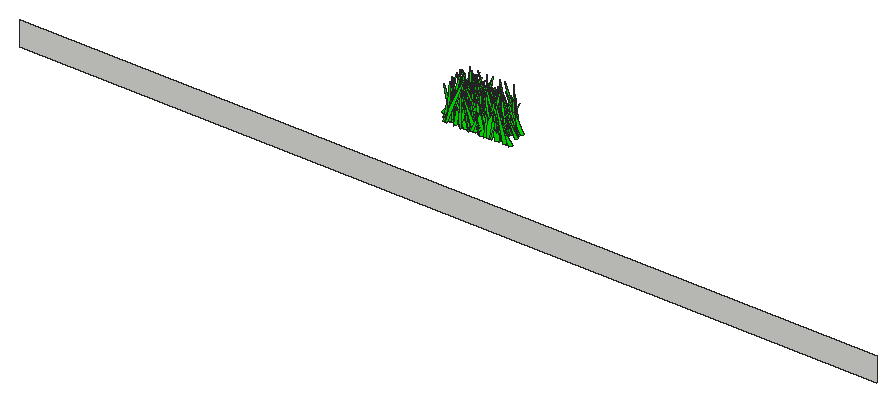
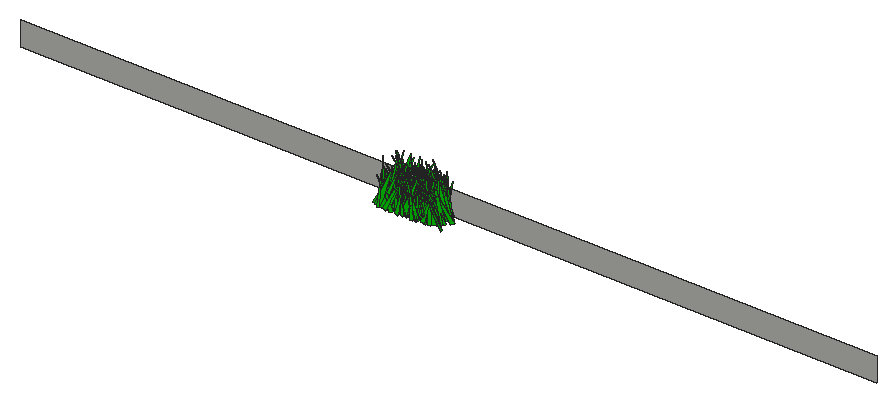
# SketchUp Ruby script. Lengths in inches.
U = 1.inch
M = Sketchup.active_model
def pt(a) = Geom::Point3d.new(a.map { |v| v * U })
def face(e, loops, mat)
  f = e.add_face(loops[0].map { |a| pt(a) })
  loops[1..].each { |l| e.add_face(l.map { |a| pt(a) }).erase! }
  f.material = f.back_material = mat if mat
  f
end
# faces: each face lists its corners as indices into pts; further lists are holes
def faces(e, pts, list, mat = nil) = list.each { |f| face(e, (f[0].is_a?(Array) ? f : [f]).map { |l| l.map { |i| pts[i] } }, mat) }
# xy, xz, yz: faces in a plane at the given z, y or x. An outline is a flat list of corners, or four numbers for a rectangle; further outlines are holes
def ring(l) = l.size == 4 ? [[l[0], l[1]], [l[2], l[1]], [l[2], l[3]], [l[0], l[3]]] : l.each_slice(2).to_a
def flat(e, list, mat, &to3) = list.each { |f| face(e, (f[0].is_a?(Array) ? f : [f]).map { |l| ring(l).map { |u, v| to3.(u, v) } }, mat) }
def xy(e, z, list, mat = nil) = flat(e, list, mat) { |x, y| [x, y, z] }
def xz(e, y, list, mat = nil) = flat(e, list, mat) { |x, z| [x, y, z] }
def yz(e, x, list, mat = nil) = flat(e, list, mat) { |y, z| [x, y, z] }
def lines(e, pts, list) = list.each { |a, b| e.add_line(pt(pts[a]), pt(pts[b])) }
# prism: a flat outline (further loops are holes) pulled along v
def prism(e, loops, v, mat = nil)
  f = face(e, loops, mat); d = Geom::Vector3d.new(v.map { |x| x * U })
  f.pushpull(f.normal.samedirection?(d) ? d.length : -d.length)
end
def box(e, o, s, mat = nil) = prism(e, [[o, [o[0] + s[0], o[1], o[2]], [o[0] + s[0], o[1] + s[1], o[2]], [o[0], o[1] + s[1], o[2]]]], [0, 0, s[2]], mat)
def at(x, y, z, deg = 0) = Geom::Transformation.translation(pt([x, y, z])) * Geom::Transformation.rotation(ORIGIN, Z_AXIS, deg.degrees)
def axes(o, x, y, z) = Geom::Transformation.new([*x, 0, *y, 0, *z, 0, *pt(o).to_a, 1])
def part(name) = M.definitions.add(name)
# library, detail: a bought-in or finely detailed component or shape, given as its bounding box
def library(name, o, s) = part(name).tap { |d| box(d.entities, o, s) }
def detail(e, o, s) = box(e.add_group.entities, o, s)
def put(e, d, t, mat = nil) = e.add_instance(d, t).tap { |i| i.material = mat if mat }
def group(e, t, mat = nil) = e.add_group.tap { |g| g.transformation = t; g.material = mat if mat }.entities
root = M.entities
M.materials.add("[0065_Lime]").color = [0, 255, 0]
c1 = part("fur_instance\#9")
p = [[0.8125,0,1.79],[0.67,-0.02,1.48],[0,-0.11,0],[0,0.11,0]]
faces(c1.entities,p,[[0,1,2,3]])
xz(root,0,[[5.71,-11.8125,282.96,-3.9375]])
put(root,c1,axes([127.84,19.68,1.48],[-1.88355,-0.98454,0.43737],[6.79232,-0.27513,-1.3991],[1.80123,0.00797,5.73327]),"[0065_Lime]")
put(root,c1,axes([127.38,20.51,1.48],[1.59601,1.1704,1.8528],[-8.58809,0.18125,1.05814],[0.89931,-0.34625,6.8167]),"[0065_Lime]")
put(root,c1,axes([130.26,19.51,1.48],[-0.54422,0.77974,1.08313],[-5.57029,-0.03175,-1.08582],[-1.23969,-0.19963,4.40342]),"[0065_Lime]")
put(root,c1,axes([130.34,19.59,1.48],[-0.93781,-0.99188,0.31196],[6.99006,-0.122,0.90495],[-1.05455,0.07338,5.721]),"[0065_Lime]")
put(root,c1,axes([128.24,18.89,1.48],[6.61511,0.29179,0.90941],[-1.22565,0.82503,-2.97163],[-2.01491,0.45612,4.79329]),"[0065_Lime]")
put(root,c1,axes([127.42,23.19,1.48],[5.41493,-0.76132,2.38586],[6.13583,0.71594,-1.55863],[-0.55627,0.48607,6.03266]),"[0065_Lime]")
put(root,c1,axes([127.24,24.58,1.48],[4.29917,0.35555,0.2939],[-2.5389,0.58261,0.95518],[0.29454,-0.16761,3.94368]),"[0065_Lime]")
put(root,c1,axes([129.75,19.5625,1.48],[4.59734,0.95656,1.01862],[-6.47828,0.66904,-1.70752],[-2.43733,0.02601,6.45982]),"[0065_Lime]")
put(root,c1,axes([127.46,20.96,1.48],[6.0247,-0.57137,1.15032],[4.28164,0.83087,-1.00807],[-0.44872,0.25659,5.8257]),"[0065_Lime]")
put(root,c1,axes([127.82,21.4375,1.48],[3.3729,-1.10577,2.71672],[8.5403,0.41349,-1.37583],[0.37891,0.52337,6.8269]),"[0065_Lime]")
put(root,c1,axes([129.15,19.16,1.48],[4.45711,-0.955,0.5882],[6.67866,0.63434,1.02719],[-1.4519,-0.01376,6.53068]),"[0065_Lime]")
put(root,c1,axes([125.68,26.09,1.48],[8.65052,0.43303,0.24417],[-3.03777,1.16273,2.10871],[0.59917,-0.35692,7.16578]),"[0065_Lime]")
put(root,c1,axes([131.32,20.62,1.48],[-0.20186,0.8961,0.26979],[-6.1799,-0.01567,-1.31541],[-1.60837,-0.05226,5.02039]),"[0065_Lime]")
put(root,c1,axes([127.74,20.66,1.48],[4.18471,0.56885,0.97148],[-4.2005,0.53816,1.4123],[0.413,-0.29038,4.52052]),"[0065_Lime]")
put(root,c1,axes([127.03,23.24,1.48],[2.50533,0.82601,1.27648],[-5.75386,0.24416,2.17777],[1.97748,-0.33608,4.71943]),"[0065_Lime]")
put(root,c1,axes([130.07,21.78,1.48],[6.79954,-0.91936,0.33816],[5.63027,0.86202,3.62678],[-3.35854,-0.41621,6.76457]),"[0065_Lime]")
put(root,c1,axes([125.55,21.65,1.48],[6.99956,-0.64941,0.12769],[4.27451,0.89339,-2.7803],[1.76403,0.41198,6.23041]),"[0065_Lime]")
put(root,c1,axes([130.36,22.59,1.48],[4.44285,-0.90294,1.68025],[6.30472,0.67925,1.20134],[-2.41016,0.11237,6.23995]),"[0065_Lime]")
put(root,c1,axes([129.98,25.67,1.48],[-3.74509,-0.71683,0.72348],[4.77236,-0.53765,-1.5054],[2.00987,-0.05907,4.92262]),"[0065_Lime]")
put(root,c1,axes([132.24,25.77,1.48],[-5.1,-0.70608,1.60563],[5.3946,-0.68136,1.29688],[0.21005,0.35533,5.67745]),"[0065_Lime]")
put(root,c1,axes([131.05,18.73,1.48],[6.55752,0.35829,2.1421],[-1.00498,0.90507,-3.03712],[-3.52512,0.40847,4.85064]),"[0065_Lime]")
put(root,c1,axes([127.3,20.04,1.48],[5.74238,1.05461,0.23828],[-7.4017,0.78577,1.48494],[1.27591,-0.18803,7.54194]),"[0065_Lime]")
put(root,c1,axes([131.45,21.28,1.48],[-7.5349,0.65973,1.91206],[-4.4009,-1.10865,1.34334],[2.86371,0.03211,7.09539]),"[0065_Lime]")
put(root,c1,axes([132.42,23.52,1.48],[3.62252,-0.92289,3.16381],[7.00436,0.64235,0.97245],[-3.03373,0.38107,6.02306]),"[0065_Lime]")
put(root,c1,axes([132.51,24.68,1.48],[-7.99573,0.44902,0.72866],[-2.3719,-1.00287,3.48749],[2.32107,0.52195,6.07398]),"[0065_Lime]")
put(root,c1,axes([135.23,25.68,1.48],[-4.03532,0.78482,0.32967],[-5.01925,-0.47578,-2.69597],[-2.4831,-0.31369,4.91378]),"[0065_Lime]")
put(root,c1,axes([131.94,25,1.48],[-8.27127,0.40188,1.98698],[-2.09799,-1.18121,2.22707],[3.12169,0.27096,6.76147]),"[0065_Lime]")
put(root,c1,axes([128.33,18.53,1.48],[8.13111,-0.63911,0.90401],[4.67579,1.1246,-1.1847],[-0.24197,0.25518,7.48517]),"[0065_Lime]")
put(root,c1,axes([131.125,19.42,1.48],[3.67897,0.90282,0.57289],[-6.32832,0.5263,-0.90377],[-1.31457,-0.00698,5.95405]),"[0065_Lime]")
put(root,c1,axes([130.91,24.08,1.48],[-3.01179,-0.78076,1.41981],[5.4629,-0.47444,-1.07506],[2.01886,0.11905,5.02715]),"[0065_Lime]")
put(root,c1,axes([132.97,19.4,1.48],[-4.59077,0.4352,1.21307],[-3.40326,-0.62465,-1.01218],[0.48395,-0.26432,4.38935]),"[0065_Lime]")
put(root,c1,axes([133.59,23.83,1.48],[-3.84347,0.70969,0.95469],[-5.16002,-0.50333,-1.20683],[-0.50961,-0.256,5.01942]),"[0065_Lime]")
put(root,c1,axes([134.07,19.27,1.48],[-2.09709,0.67834,0.34016],[-4.55195,-0.25384,-1.60503],[-1.66105,-0.16079,3.96898]),"[0065_Lime]")
put(root,c1,axes([133.15,19.125,1.48],[-5.94132,0.15971,0.73819],[-0.86372,-0.81893,1.33753],[1.17021,0.20643,4.7351]),"[0065_Lime]")
put(root,c1,axes([132.39,21.64,1.48],[6.24431,-0.53352,1.84624],[2.8622,0.90798,2.38724],[-3.37273,-0.21722,5.44403]),"[0065_Lime]")
put(root,c1,axes([131.27,23.78,1.48],[7.11686,0.5597,1.48646],[-3.72566,1.03061,-1.20132],[-2.30748,0.06225,6.52426]),"[0065_Lime]")
put(root,c1,axes([130.68,19.57,1.48],[7.94743,0.52318,0.88197],[-3.31714,1.09713,-2.03117],[-2.00871,0.25819,6.84374]),"[0065_Lime]")
put(root,c1,axes([129.43,24.15,1.48],[8.37788,-0.04501,0.69259],[0.48877,1.15748,-1.39106],[-0.76727,0.24584,6.67627]),"[0065_Lime]")
put(root,c1,axes([131.43,18.84,1.48],[6.79196,0.75194,0.95465],[-5.00898,0.95874,-1.72581],[-2.2188,0.13739,6.81835]),"[0065_Lime]")
put(root,c1,axes([129.02,24.9,1.48],[0.3596,-1.28657,0.19297],[8.49208,0.03434,-2.79914],[3.4311,0.04986,6.90773]),"[0065_Lime]")
put(root,c1,axes([133.03,24.78,1.48],[1.52368,-0.62606,0.68471],[4.2637,0.24029,1.0844],[-1.54267,0.04576,3.67341]),"[0065_Lime]")
put(root,c1,axes([133.73,24.19,1.48],[-2.94012,0.67888,1.28121],[-5.07695,-0.38151,-0.93462],[-0.21714,-0.27226,4.5044]),"[0065_Lime]")
put(root,c1,axes([131.56,25.58,1.48],[5.7235,0.63245,0.26773],[-4.17912,0.77098,-1.91723],[-1.70327,0.23356,5.60375]),"[0065_Lime]")
put(root,c1,axes([133.91,26.06,1.48],[-7.40548,-0.24155,1.73235],[2.13299,-1.05028,1.12575],[1.71492,0.26327,6.08053]),"[0065_Lime]")
put(root,c1,axes([134.16,19.74,1.48],[-5.31076,0.24298,0.03166],[-1.63072,-0.7093,1.42198],[0.57639,0.23198,4.31477]),"[0065_Lime]")
put(root,c1,axes([131.96,22.92,1.48],[-1.17886,0.83181,1.0892],[-5.88421,-0.2036,0.99651],[1.4868,-0.14626,4.80742]),"[0065_Lime]")
put(root,c1,axes([132.56,24.0625,1.48],[-2.37055,0.96935,0.27023],[-6.76377,-0.33583,1.10872],[1.39646,0.01894,5.82882]),"[0065_Lime]")
put(root,c1,axes([134.84,18.94,1.48],[-3.13554,0.64764,0.29956],[-4.55574,-0.42207,-0.97376],[-0.78964,-0.13661,4.42852]),"[0065_Lime]")
put(root,c1,axes([130.73,19.98,1.48],[1.56005,-0.66734,0.73],[4.53678,0.1565,-1.62082],[1.6665,0.19866,3.72907]),"[0065_Lime]")
put(root,c1,axes([132.38,19.88,1.48],[-4.58927,0.68722,1.07387],[-4.29088,-0.66041,2.02906],[2.69252,0.11889,5.06393]),"[0065_Lime]")
put(root,c1,axes([129.71,23.44,1.48],[6.23921,0.88257,0.74493],[-6.29047,0.8357,1.68191],[0.84722,-0.29463,7.00204]),"[0065_Lime]")
put(root,c1,axes([130.44,21.64,1.48],[8.73592,0.02809,1.0369],[-0.69268,1.13637,2.82962],[-1.08864,-0.49762,6.52025]),"[0065_Lime]")
put(root,c1,axes([131.79,22.34,1.48],[5.87142,0.09701,0.89122],[-0.36134,0.80914,-1.3762],[-1.24358,0.22291,4.60766]),"[0065_Lime]")
put(root,c1,axes([131.51,22.72,1.48],[2.46936,-0.62367,0.64679],[4.41968,0.30954,-1.16271],[0.89336,0.19254,3.96441]),"[0065_Lime]")
put(root,c1,axes([130.8,24.49,1.48],[5.97716,-0.62244,1.40996],[4.75421,0.76903,-1.95864],[0.15444,0.41634,5.72576]),"[0065_Lime]")
put(root,c1,axes([136.28,19.59,1.48],[-2.50424,-0.58005,0.30026],[3.56717,-0.27082,2.15339],[-2.10991,0.2306,3.2843]),"[0065_Lime]")
put(root,c1,axes([135.14,25.03,1.48],[1.04984,0.83458,1.67244],[-5.80698,0.24086,-1.61581],[-2.40459,-0.2173,4.63229]),"[0065_Lime]")
put(root,c1,axes([133.13,18.63,1.48],[-4.8097,-0.56357,1.36731],[3.48379,-0.71014,-1.69983],[2.60272,-0.09091,4.80199]),"[0065_Lime]")
put(root,c1,axes([133.46,23.15,1.48],[4.6814,0.82059,0.23858],[-5.52111,0.63774,-1.82309],[-1.92513,0.16646,5.80864]),"[0065_Lime]")
put(root,c1,axes([132.64,24.52,1.48],[5.42971,-0.40406,0.14494],[2.72941,0.73854,1.33857],[-0.9222,-0.19315,4.81511]),"[0065_Lime]")
put(root,c1,axes([136.28,24.37,1.48],[-5.68369,0.11795,0.29079],[-0.90555,-0.76792,-1.27349],[0.1111,-0.22512,4.49647]),"[0065_Lime]")
put(root,c1,axes([134.37,25.72,1.48],[-3.44311,-0.5649,0.56146],[3.80648,-0.4906,-1.09557],[1.46586,-0.05291,4.16373]),"[0065_Lime]")
put(root,c1,axes([131.8,21.55,1.48],[3.70211,-1.08959,0.22756],[7.67112,0.50743,-1.15718],[1.16561,0.12116,6.89284]),"[0065_Lime]")
put(root,c1,axes([134.05,24.375,1.48],[6.28003,-0.35878,2.98637],[3.7125,0.91411,-1.4855],[-2.49312,0.45747,5.31045]),"[0065_Lime]")
put(root,c1,axes([135.52,20.25,1.48],[-7.56193,0.32921,1.29869],[-1.80756,-1.05216,1.97363],[2.18419,0.26903,6.12951]),"[0065_Lime]")
put(root,c1,axes([131.31,20.84,1.48],[8.74302,0.23964,0.05454],[-1.65699,1.2036,-1.46434],[-0.40912,0.24653,7.09621]),"[0065_Lime]")
put(root,c1,axes([134.72,22.1,1.48],[5.09673,-0.77492,1.57839],[5.32278,0.7647,1.20829],[-2.41775,0.04996,5.98742]),"[0065_Lime]")
put(root,c1,axes([133.23,18.88,1.48],[7.89269,-0.3569,2.56838],[3.54797,1.07796,-2.19447],[-1.95783,0.51467,6.37725]),"[0065_Lime]")
put(root,c1,axes([137.68,22.93,1.48],[-5.83603,-0.4904,0.36089],[3.45664,-0.77685,1.61127],[-0.65455,0.27001,5.29127]),"[0065_Lime]")
put(root,c1,axes([137.08,24.58,1.48],[-3.639,0.53306,1.42163],[-4.09878,-0.39308,-2.00284],[-0.8036,-0.40899,3.77784]),"[0065_Lime]")
put(root,c1,axes([133.62,24.89,1.48],[6.8678,-0.07761,1.28988],[0.21147,0.9707,1.21212],[-1.66582,-0.19674,5.47175]),"[0065_Lime]")
put(root,c1,axes([136,18.625,1.48],[-4.96977,-0.14821,1.25753],[1.45572,-0.69353,1.06749],[1.17619,0.23213,3.99226]),"[0065_Lime]")
put(root,c1,axes([137.1,25.68,1.48],[-8.70175,-0.25326,0.94629],[1.23958,-1.15103,-2.78079],[1.7508,-0.44381,6.67205]),"[0065_Lime]")
put(root,c1,axes([133.01,19.67,1.48],[4.3497,-0.27401,0.18043],[1.90095,0.56937,-1.34642],[0.48806,0.22443,3.63611]),"[0065_Lime]")
put(root,c1,axes([136.52,20.64,1.48],[-6.98711,-0.41337,0.98387],[2.65637,-0.984,-1.37157],[1.74944,-0.15684,6.01213]),"[0065_Lime]")
put(root,c1,axes([135.93,19.75,1.48],[2.51291,-0.7947,0.59097],[5.3811,0.36742,1.41693],[-1.8859,-0.01055,4.83042]),"[0065_Lime]")
put(root,c1,axes([135.55,22.21,1.48],[-6.97969,0.72171,2.2043],[-5.02118,-1.04913,0.99068],[2.91733,-0.07903,6.97888]),"[0065_Lime]")
put(root,c1,axes([134.34,23.32,1.48],[6.02519,0.46674,0.69826],[-3.03176,0.83849,-1.47195],[-1.60571,0.16823,5.39932]),"[0065_Lime]")
put(root,c1,axes([137.44,21.26,1.48],[-4.47893,-0.43545,1.21376],[3.42862,-0.53799,1.9036],[-0.27257,0.38812,4.0004]),"[0065_Lime]")
put(root,c1,axes([136.15,22.61,1.48],[-5.37648,-0.31735,1.10742],[2.00376,-0.77406,-0.99633],[1.71433,-0.09052,4.63764]),"[0065_Lime]")
put(root,c1,axes([133.04,22.99,1.48],[8.93321,-0.06221,0.97484],[0.20968,1.24475,1.39025],[-1.26028,-0.23383,7.14124]),"[0065_Lime]")
put(root,c1,axes([133.65,25.9,1.48],[6.77364,-0.5246,1.84911],[4.26715,0.92129,-1.58402],[-0.94702,0.39901,6.08853]),"[0065_Lime]")
put(root,c1,axes([135.52,24.7,1.48],[-5.21227,0.12291,2.40316],[-1.87487,-0.77391,-1.36424],[2.44508,-0.33143,4.07681]),"[0065_Lime]")
put(root,c1,axes([135.08,26.47,1.48],[-5.39802,-0.85143,1.97427],[5.76655,-0.82942,-1.55414],[3.05819,0.06109,6.41528]),"[0065_Lime]")
put(root,c1,axes([137.76,25.1875,1.48],[-1.08888,-0.92728,0.02245],[6.32522,-0.14553,1.55459],[-1.8814,0.04739,5.21348]),"[0065_Lime]")
put(root,c1,axes([134.4,24.15,1.48],[-1.71185,1.06034,0.21618],[-7.21689,-0.24103,1.8036],[2.21998,0.03408,6.02997]),"[0065_Lime]")
put(root,c1,axes([134.83,25.73,1.48],[-1.10419,0.69693,0.40557],[-4.75332,-0.16882,1.15867],[1.5011,-0.02194,3.96733]),"[0065_Lime]")
put(root,c1,axes([135.82,18.75,1.48],[-7.96727,0.39788,1.93141],[-1.08809,-1.01041,4.00505],[3.5315,0.58631,5.59137]),"[0065_Lime]")
put(root,c1,axes([139.39,19.86,1.48],[-9.31701,-0.11263,0.27871],[0.84257,-1.29607,1.08597],[0.22337,0.19112,7.52865]),"[0065_Lime]")
put(root,c1,axes([137.85,18.92,1.48],[-0.79557,-1.00982,0.39914],[6.98197,-0.09105,1.48901],[-1.7714,0.09467,5.68964]),"[0065_Lime]")
put(root,c1,axes([134.58,23.68,1.48],[0.74397,-0.7004,1.1461],[5.03176,0.05025,-1.13211],[1.22942,0.21818,3.93991]),"[0065_Lime]")
put(root,c1,axes([138.53,25.48,1.48],[-0.88903,1.15703,2.31859],[-8.36816,-0.00115,-2.10376],[-2.42875,-0.41956,6.39972]),"[0065_Lime]")
put(root,c1,axes([135.64,18.93,1.48],[5.81527,0.43002,0.63539],[-2.33113,0.73955,-2.65563],[-2.13104,0.36447,4.63886]),"[0065_Lime]")
put(root,c1,axes([134.18,19.3,1.48],[-0.80773,1.07207,0.55989],[-7.15448,-0.14033,2.17514],[2.73783,-0.05043,5.84924]),"[0065_Lime]")
put(root,c1,axes([138.44,24.83,1.48],[-4.54121,0.92378,0.97055],[-6.67581,-0.61892,-0.92706],[-0.27693,-0.22857,6.43281]),"[0065_Lime]")
put(root,c1,axes([134.27,19.71,1.48],[0.97731,-0.92421,1.43279],[6.52881,0.05621,-1.73162],[1.93307,0.27742,5.12403]),"[0065_Lime]")
put(root,c1,axes([134.97,25.71,1.48],[4.5144,0.95282,2.04613],[-7.22708,0.61018,1.02867],[-0.27541,-0.39373,6.54579]),"[0065_Lime]")
put(root,c1,axes([132.75,21.7,1.48],[5.23452,0.91555,0.72028],[-6.24935,0.64323,2.6518],[2.04506,-0.37783,6.25982]),"[0065_Lime]")
put(root,c1,axes([134.63,19.55,1.48],[-0.24559,-0.95133,0.45507],[6.30165,-0.06128,-2.04286],[2.53719,0.06013,5.11792]),"[0065_Lime]")
put(root,c1,axes([133.75,22.38,1.48],[3.68483,0.64414,0.29703],[-4.17564,0.44113,2.21775],[1.92642,-0.27593,4.23897]),"[0065_Lime]")
put(root,c1,axes([137.39,19.5,1.48],[-4.49399,-0.57491,0.29517],[3.77762,-0.60818,-1.63968],[1.6126,-0.17744,4.66361]),"[0065_Lime]")
put(root,c1,axes([136.86,19.7,1.48],[-3.35789,-0.93117,0.86434],[6.44768,-0.49393,-1.25741],[1.86274,0.03109,5.9105]),"[0065_Lime]")
put(root,c1,axes([137.45,23.86,1.48],[4.04449,0.2949,1.45767],[-1.7789,0.62016,-0.93846],[-2.10982,0.04243,3.58559]),"[0065_Lime]")
put(root,c1,axes([139.39,23.59,1.48],[-0.38066,0.95956,0.82046],[-6.53336,-0.00427,-1.83842],[-2.22805,-0.15143,5.25066]),"[0065_Lime]")
put(root,c1,axes([140.41,19.68,1.48],[-3.81682,-1.17339,0.18233],[8.1746,-0.51753,1.61864],[-1.71942,0.14424,7.29076]),"[0065_Lime]")
put(root,c1,axes([135.63,24.29,1.48],[7.39248,0.11661,0.85523],[-0.49729,1.00837,-1.76322],[-1.24373,0.28994,5.78832]),"[0065_Lime]")
put(root,c1,axes([137.21,20.5,1.48],[4.76854,-0.84726,0.64072],[5.83598,0.67718,1.26846],[-1.70801,-0.05163,6.12294]),"[0065_Lime]")
put(root,c1,axes([134.48,21.66,1.48],[4.83598,0.94025,0.77104],[-6.61859,0.62582,1.89338],[1.36624,-0.29642,6.44306]),"[0065_Lime]")
put(root,c1,axes([135.54,22.1,1.48],[7.36135,-0.15432,0.40554],[0.74953,0.92479,2.79049],[-0.94495,-0.46868,5.37264]),"[0065_Lime]")
put(root,c1,axes([141.89,19.29,1.48],[-4.31449,0.84538,0.19195],[-5.47768,-0.53421,-2.62402],[-2.49906,-0.28856,5.42021]),"[0065_Lime]")
put(root,c1,axes([138.77,19,1.48],[-8.73321,0.07854,2.45287],[0.45658,-1.23132,2.39663],[3.03271,0.41154,6.70265]),"[0065_Lime]")
put(root,c1,axes([140.08,21.92,1.48],[-2.22002,-0.79884,1.11367],[5.71154,-0.25211,1.47338],[-1.25361,0.26602,4.74061]),"[0065_Lime]")
put(root,c1,axes([137.24,23.71,1.48],[5.57201,0.38544,0.24966],[-2.28169,0.69791,-2.41171],[-1.55306,0.35751,4.43891]),"[0065_Lime]")
put(root,c1,axes([138.86,22.95,1.48],[-6.83398,-0.10005,1.84405],[-0.32981,-0.92065,-2.48244],[2.35323,-0.41958,5.00737]),"[0065_Lime]")
put(root,c1,axes([136.65,21.56,1.48],[7.90089,-0.47074,0.74765],[2.9411,1.07722,2.1632],[-1.84865,-0.29808,6.63689]),"[0065_Lime]")
put(root,c1,axes([136.09,23.33,1.48],[1.00671,1.08879,0.60948],[-7.54191,0.11012,1.65064],[1.92836,-0.13774,6.13753]),"[0065_Lime]")
put(root,c1,axes([140.23,22.48,1.48],[-8.05617,0.19328,1.51644],[-1.82605,-1.11309,-1.66452],[1.42591,-0.33341,6.43606]),"[0065_Lime]")
put(root,c1,axes([134.81,22.43,1.48],[6.21566,-0.63499,0.30436],[4.37164,0.81549,-2.05835],[1.20404,0.31714,5.90225]),"[0065_Lime]")
put(root,c1,axes([136.18,21.36,1.48],[6.63995,0.13353,0.02442],[-0.88233,0.87652,-1.87333],[-0.3542,0.3198,5.12437]),"[0065_Lime]")
put(root,c1,axes([136.92,18.75,1.48],[5.36441,-0.29738,0.86585],[2.31962,0.73454,-1.05512],[-0.48075,0.2259,4.57055]),"[0065_Lime]")
put(root,c1,axes([139.23,20.37,1.48],[2.75928,0.98315,0.51912],[-6.80064,0.39795,-1.33775],[-1.7639,0.00368,5.96968]),"[0065_Lime]")
put(root,c1,axes([138.42,21.66,1.48],[5.12043,0.83118,0.14475],[-5.60115,0.69137,-1.93495],[-1.90996,0.20082,6.06248]),"[0065_Lime]")
put(root,c1,axes([139.67,21.8125,1.48],[-4.72857,0.40873,2.00454],[-3.61637,-0.65552,-1.1654],[1.2066,-0.3629,4.36278]),"[0065_Lime]")
put(root,c1,axes([138.625,26.1,1.48],[3.80662,-0.40922,0.0005],[2.51978,0.46289,1.95396],[-1.46003,-0.26805,3.37354]),"[0065_Lime]")
put(root,c1,axes([137.92,25.57,1.48],[4.73747,-0.20897,0.45323],[1.15431,0.62229,1.63117],[-1.09071,-0.24909,3.69489]),"[0065_Lime]")
put(root,c1,axes([141.32,22.24,1.48],[-1.17097,-0.75998,0.3781],[5.02305,-0.12636,1.78183],[-2.05816,0.12399,4.13351]),"[0065_Lime]")
put(root,c1,axes([140.54,20.18,1.48],[-6.95039,0.78364,2.46634],[-6.18035,-0.97956,-1.09437],[1.44842,-0.41934,7.16537]),"[0065_Lime]")
put(root,c1,axes([140.41,18.56,1.48],[0.4911,1.11012,1.31598],[-7.88306,0.11408,-1.27832],[-1.69933,-0.2084,6.31034]),"[0065_Lime]")
put(root,c1,axes([137.55,19.06,1.48],[0.86224,-0.64256,0.8948],[4.48378,0.06485,-1.29813],[1.42002,0.18539,3.55557]),"[0065_Lime]")
put(root,c1,axes([138.75,21.75,1.48],[-3.1877,0.67167,0.07836],[-4.34556,-0.41384,1.90088],[1.99334,0.17193,4.26932]),"[0065_Lime]")
put(root,c1,axes([136.91,22.09,1.48],[4.09646,0.48413,0.08719],[-3.36276,0.55615,1.0575],[0.7574,-0.14924,4.22357]),"[0065_Lime]")
put(root,c1,axes([140.09,26.51,1.48],[1.98822,-0.64215,0.26388],[4.26198,0.27748,1.37997],[-1.68065,-0.056,3.81166]),"[0065_Lime]")
put(root,c1,axes([139.0625,20.37,1.48],[7.74609,-0.26556,2.07598],[0.64318,1.05701,2.94288],[-3.1099,-0.44283,5.77947]),"[0065_Lime]")
put(root,c1,axes([141.26,19.45,1.48],[-3.26171,-0.59841,0.96391],[4.39806,-0.41853,1.14017],[-0.44413,0.25026,4.2117]),"[0065_Lime]")
put(root,c1,axes([142,19.49,1.48],[-2.60916,0.84943,0.55889],[-5.924,-0.33079,-1.45191],[-1.38563,-0.18526,5.15497]),"[0065_Lime]")
put(root,c1,axes([139.14,25.75,1.48],[6.16351,-0.46399,1.36798],[3.03194,0.89513,1.13527],[-2.1305,-0.06845,5.57317]),"[0065_Lime]")
put(root,c1,axes([141.14,21.84,1.48],[1.10791,-0.59627,2.17495],[4.60674,0.27314,0.95656],[-1.98339,0.30133,3.43669]),"[0065_Lime]")
put(root,c1,axes([140.32,25.64,1.48],[-3.72223,0.22275,0.77798],[-1.22082,-0.52218,1.14538],[1.3919,0.13769,3.0851]),"[0065_Lime]")
put(root,c1,axes([138.61,25.48,1.48],[7.21011,-0.22965,0.99704],[1.21499,0.98998,1.82754],[-1.64234,-0.27583,5.72915]),"[0065_Lime]")
put(root,c1,axes([138.64,21.71,1.48],[6.75246,0.3121,1.58934],[-2.63049,0.94651,1.16614],[-1.35337,-0.28249,5.66323]),"[0065_Lime]")
put(root,c1,axes([140.16,19.76,1.48],[-3.36448,0.87015,0.77132],[-6.04919,-0.49057,1.08663],[1.62889,-0.02454,5.62856]),"[0065_Lime]")
put(root,c1,axes([142.56,24.83,1.48],[-8.44716,0.09438,1.51118],[-1.48844,-1.05783,-3.29101],[1.29893,-0.59838,6.0563]),"[0065_Lime]")
put(root,c1,axes([140.88,24.88,1.48],[-5.85032,0.45389,1.19981],[-2.79656,-0.83509,1.5638],[2.18831,0.14624,5.2061]),"[0065_Lime]")
put(root,c1,axes([142.27,21.5625,1.48],[-2.92992,-0.66664,1.19128],[4.95046,-0.37391,1.04441],[-0.38062,0.26841,4.41369]),"[0065_Lime]")
put(root,c1,axes([139.5625,22.9,1.48],[5.06555,-0.14829,0.54054],[0.89635,0.70451,0.91839],[-0.86705,-0.13801,4.10742]),"[0065_Lime]")
put(root,c1,axes([135.55,20.67,1.48],[7.21784,0.82875,0.21409],[-5.256,0.87546,3.68372],[2.68852,-0.51343,6.62681]),"[0065_Lime]")
put(root,c1,axes([139.24,21.55,1.48],[2.58422,-0.4432,0.34814],[3.0906,0.33086,-1.0648],[0.76125,0.16128,3.14116]),"[0065_Lime]")
put(root,c1,axes([142.18,23.9,1.48],[-5.66061,-0.45991,0.35499],[2.98111,-0.76416,-1.72256],[1.41984,-0.22914,5.03202]),"[0065_Lime]")
put(root,c1,axes([137.94,22.84,1.48],[6.64987,0.45998,0.20258],[-3.22452,0.90032,1.53242],[0.61639,-0.25259,5.83093]),"[0065_Lime]")
put(root,c1,axes([140.37,23.29,1.48],[5.39388,0.28564,0.77653],[-1.74858,0.75316,-1.2473],[-1.40927,0.15877,4.51974]),"[0065_Lime]")
put(root,c1,axes([138.82,18.92,1.48],[5.44508,0.27023,0.14529],[-1.90623,0.73986,1.15688],[0.31064,-0.19664,4.55253]),"[0065_Lime]")
put(root,c1,axes([140.67,25.5,1.48],[-1.8538,-0.77308,0.65667],[5.33423,-0.28101,-1.12221],[1.57038,0.04192,4.58707]),"[0065_Lime]")
put(root,c1,axes([143.52,25.49,1.48],[-6.02181,-0.37426,0.67955],[2.77549,-0.83253,0.90876],[0.29742,0.19152,5.27829]),"[0065_Lime]")
put(root,c1,axes([143.35,22.98,1.48],[-4.19326,-0.98526,1.86504],[7.37029,-0.54369,1.33964],[-0.3154,0.3942,6.50905]),"[0065_Lime]")
put(root,c1,axes([142.875,20.14,1.48],[-2.05655,0.88896,1.18098],[-6.45927,-0.25924,-0.90347],[-0.63862,-0.24068,5.33501]),"[0065_Lime]")
put(root,c1,axes([143.21,26.16,1.48],[-1.03097,0.62335,1.15789],[-4.4184,-0.06585,-1.41503],[-1.47749,-0.23804,3.42364]),"[0065_Lime]")
put(root,c1,axes([139.99,22.39,1.48],[6.82384,0.04362,0.98574],[-0.55605,0.9517,1.13562],[-1.12061,-0.20661,5.43905]),"[0065_Lime]")
put(root,c1,axes([142.9,20.64,1.48],[-6.82891,0.45378,1.02786],[-2.9265,-0.96451,1.40429],[1.86042,0.14845,5.98189]),"[0065_Lime]")
put(root,c1,axes([141.36,18.53,1.48],[4.23079,-0.34781,0.45628],[2.16617,0.57471,1.3902],[-1.32246,-0.17134,3.73684]),"[0065_Lime]")
put(root,c1,axes([140.41,20.36,1.48],[2.02059,-0.67807,1.2145],[4.97355,0.22759,-1.21696],[0.88252,0.26988,4.07764]),"[0065_Lime]")
put(root,c1,axes([144.8,20.48,1.48],[-0.45692,1.13544,3.53501],[-8.71408,0.13765,-2.22679],[-2.87145,-0.59841,6.19519]),"[0065_Lime]")
put(root,c1,axes([142.71,19.18,1.48],[6.75,-0.5458,2.59236],[3.32885,1.0476,1.65588],[-3.76333,-0.0523,6.11442]),"[0065_Lime]")
put(root,c1,axes([145.55,25.3,1.48],[-4.95574,-0.71628,0.20309],[4.87261,-0.64951,1.90722],[-1.5179,0.25355,5.45931]),"[0065_Lime]")
put(root,c1,axes([144.01,26.34,1.48],[-2.16657,-0.66253,0.06643],[4.6074,-0.29472,0.92883],[-1.00445,0.07718,4.11722]),"[0065_Lime]")
put(root,c1,axes([145.09,25.92,1.48],[-5.73431,0.64906,1.05107],[-4.79538,-0.77001,-1.37646],[-0.09838,-0.29886,5.82908]),"[0065_Lime]")
put(root,c1,axes([142.13,21.46,1.48],[3.95981,0.57581,0.21533],[-3.9433,0.54764,-1.09234],[-1.14552,0.10527,4.50461]),"[0065_Lime]")
put(root,c1,axes([145.3,23.31,1.48],[-8.4659,-0.4315,0.21637],[2.89354,-1.15024,-1.9577],[1.062,-0.30578,7.05884]),"[0065_Lime]")
put(root,c1,axes([144.83,19.15,1.48],[2.98002,1.15766,2.56783],[-8.06763,0.54708,-2.06991],[-3.57111,-0.26987,6.81903]),"[0065_Lime]")
put(root,c1,axes([141.69,18.61,1.48],[-1.71639,1.03221,1.25902],[-7.21186,-0.28867,1.42551],[2.08462,-0.1488,5.96823]),"[0065_Lime]")
put(root,c1,axes([147.82,19.63,1.48],[-3.7905,0.80269,0.18062],[-4.59833,-0.40586,-3.40874],[-3.39651,-0.34633,4.41331]),"[0065_Lime]")
put(root,c1,axes([144.72,19.6,1.48],[-4.85139,-0.10869,0.78537],[1.04932,-0.65236,1.26339],[0.65534,0.23992,3.79105]),"[0065_Lime]")
put(root,c1,axes([141.95,26.32,1.48],[0.25823,-0.78712,0.21291],[5.39769,0.02491,-1.24602],[1.52029,0.04527,4.38776]),"[0065_Lime]")
put(root,c1,axes([145.41,23.68,1.48],[-8.94362,-0.22783,1.97823],[2.24673,-1.23953,1.93713],[1.86966,0.39969,7.13515]),"[0065_Lime]")
put(root,c1,axes([142.3,20.23,1.48],[8.56276,0.23459,1.86934],[-1.42136,1.24186,-0.91445],[-2.45934,0.09906,7.03704]),"[0065_Lime]")
put(root,c1,axes([142.82,23.54,1.48],[5.24919,0.33066,0.54928],[-1.98267,0.70588,-1.70269],[-1.43612,0.23409,4.35838]),"[0065_Lime]")
put(root,c1,axes([142.35,19,1.48],[0.39854,1.2719,0.75248],[-8.99165,0.03516,1.15953],[1.39135,-0.1371,7.27796]),"[0065_Lime]")
put(root,c1,axes([140.78,23.125,1.48],[5.04298,0.76972,0.06193],[-5.36768,0.69134,1.26677],[1.09538,-0.15592,5.92243]),"[0065_Lime]")
put(root,c1,axes([139.6,20.43,1.48],[3.90092,0.84715,0.34499],[-5.21328,0.43578,3.14475],[3.05739,-0.3378,4.92208]),"[0065_Lime]")
put(root,c1,axes([146.37,23.8,1.48],[-4.09029,-1.07044,0.48089],[7.60214,-0.56068,0.96163],[-0.76695,0.15127,6.96711]),"[0065_Lime]")
put(root,c1,axes([146.64,25.76,1.48],[-1.46831,1.22973,0.40451],[-8.47423,-0.18103,-1.91093],[-2.24118,-0.12117,6.9605]),"[0065_Lime]")
put(root,c1,axes([142.125,18.83,1.48],[6.98412,-0.37282,1.87956],[3.37004,0.91622,-2.19553],[-1.01083,0.47865,5.66664]),"[0065_Lime]")
put(root,c1,axes([144.5,19.4375,1.48],[-4.00532,-0.59415,0.22775],[3.95155,-0.54324,-1.50847],[1.53044,-0.15234,4.4909]),"[0065_Lime]")
put(root,c1,axes([145.5,21.01,1.48],[-0.39016,-0.89065,0.56664],[6.27232,-0.03595,0.96419],[-1.14817,0.10628,5.07469]),"[0065_Lime]")
put(root,c1,axes([144.23,24.08,1.48],[-3.12516,0.84391,1.09383],[-5.87944,-0.47202,1.08891],[1.81922,-0.07579,5.39824]),"[0065_Lime]")
put(root,c1,axes([145.62,21.28,1.48],[-6.65893,0.71906,0.08223],[-4.74503,-0.87604,2.4612],[1.91862,0.32908,6.37232]),"[0065_Lime]")
put(root,c1,axes([145.66,21.5,1.48],[-8.33006,0.04661,2.46563],[-1.42991,-1.15412,-2.46518],[2.69327,-0.46857,6.31719]),"[0065_Lime]")
put(root,c1,axes([142.58,25.37,1.48],[5.76767,-0.11747,0.32869],[0.90169,0.79389,-0.9609],[-0.22174,0.17265,4.64212]),"[0065_Lime]")
put(root,c1,axes([147.61,24.6,1.48],[-5.011,-0.32905,0.21449],[2.28979,-0.65933,1.50072],[-0.55677,0.24992,4.24145]),"[0065_Lime]")
put(root,c1,axes([147.91,25.4,1.48],[-5.18575,0.70814,0.36892],[-5.00649,-0.70487,-1.22478],[-0.73331,-0.19547,5.75295]),"[0065_Lime]")
put(root,c1,axes([146.11,19.93,1.48],[-6.34502,0.55421,0.71581],[-3.59095,-0.87884,1.74044],[1.85347,0.19457,5.82241]),"[0065_Lime]")
put(root,c1,axes([143.62,24.0625,1.48],[1.54337,-0.68788,0.84582],[4.86756,0.1708,-1.22201],[1.16294,0.19802,3.9923]),"[0065_Lime]")
put(root,c1,axes([147.79,23.52,1.48],[-6.87355,0.26782,0.67526],[-2.02604,-0.95329,-0.97559],[0.46594,-0.19423,5.7194]),"[0065_Lime]")
put(root,c1,axes([146.61,24.71,1.48],[-4.90062,0.56025,0.21152],[-3.88573,-0.68175,0.94241],[0.93008,0.10372,5.05168]),"[0065_Lime]")
put(root,c1,axes([149.35,19.04,1.48],[-4.25283,0.82828,0.03249],[-5.41189,-0.5459,-2.36475],[-2.33624,-0.2432,5.41881]),"[0065_Lime]")
put(root,c1,axes([146.75,24.25,1.48],[0.32569,-0.80501,1.67459],[5.92412,0.10859,0.98695],[-1.4012,0.27201,4.56194]),"[0065_Lime]")
put(root,c1,axes([147.7,18.77,1.48],[-6.10664,-0.84118,2.02582],[6.46,-0.83044,1.32946],[0.55402,0.41129,6.82762]),"[0065_Lime]")
put(root,c1,axes([145.98,26.45,1.48],[-5.71622,-0.6116,0.9142],[3.85744,-0.79855,-1.94309],[2.30807,-0.18008,5.51159]),"[0065_Lime]")
put(root,c1,axes([145.62,18.98,1.48],[4.37142,0.2803,0.81749],[-1.49199,0.59741,-1.5851],[-1.66223,0.20092,3.57263]),"[0065_Lime]")
put(root,c1,axes([143.4,19.99,1.48],[2.30373,0.65556,0.49754],[-4.35928,0.26135,1.81598],[1.77095,-0.20947,3.8229]),"[0065_Lime]")
put(root,c1,axes([146.27,23.93,1.48],[6.95389,0.8112,1.9267],[-5.2322,1.02957,-2.03086],[-3.40019,0.07473,7.06545]),"[0065_Lime]")
put(root,c1,axes([148.12,22.93,1.48],[-2.78802,-0.67224,0.26662],[4.68608,-0.37065,1.10656],[-1.01744,0.13499,4.36596]),"[0065_Lime]")
